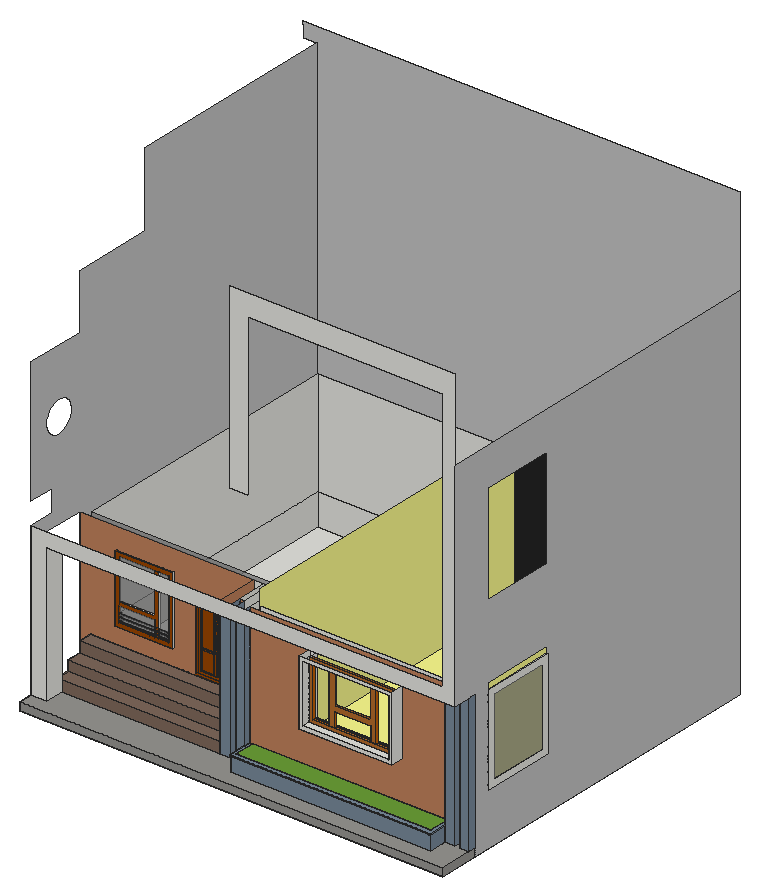
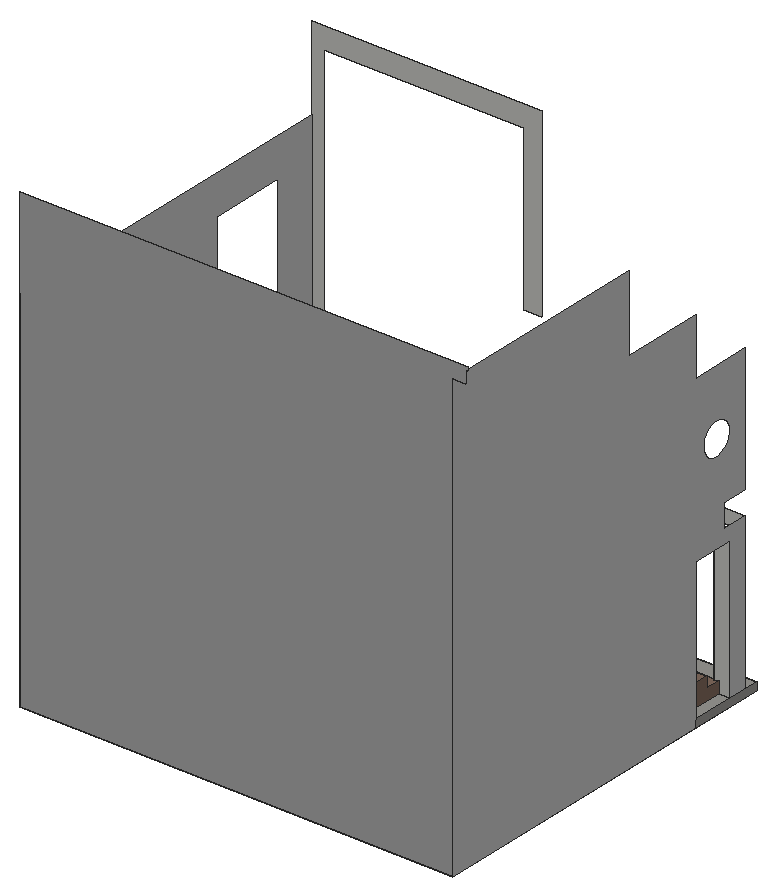
# SketchUp Ruby script. Lengths in inches.
U = 1.inch
M = Sketchup.active_model
def pt(a) = Geom::Point3d.new(a.map { |v| v * U })
def face(e, loops, mat)
  f = e.add_face(loops[0].map { |a| pt(a) })
  loops[1..].each { |l| e.add_face(l.map { |a| pt(a) }).erase! }
  f.material = f.back_material = mat if mat
  f
end
# faces: each face lists its corners as indices into pts; further lists are holes
def faces(e, pts, list, mat = nil) = list.each { |f| face(e, (f[0].is_a?(Array) ? f : [f]).map { |l| l.map { |i| pts[i] } }, mat) }
# xy, xz, yz: faces in a plane at the given z, y or x. An outline is a flat list of corners, or four numbers for a rectangle; further outlines are holes
def ring(l) = l.size == 4 ? [[l[0], l[1]], [l[2], l[1]], [l[2], l[3]], [l[0], l[3]]] : l.each_slice(2).to_a
def flat(e, list, mat, &to3) = list.each { |f| face(e, (f[0].is_a?(Array) ? f : [f]).map { |l| ring(l).map { |u, v| to3.(u, v) } }, mat) }
def xy(e, z, list, mat = nil) = flat(e, list, mat) { |x, y| [x, y, z] }
def xz(e, y, list, mat = nil) = flat(e, list, mat) { |x, z| [x, y, z] }
def yz(e, x, list, mat = nil) = flat(e, list, mat) { |y, z| [x, y, z] }
def lines(e, pts, list) = list.each { |a, b| e.add_line(pt(pts[a]), pt(pts[b])) }
# prism: a flat outline (further loops are holes) pulled along v
def prism(e, loops, v, mat = nil)
  f = face(e, loops, mat); d = Geom::Vector3d.new(v.map { |x| x * U })
  f.pushpull(f.normal.samedirection?(d) ? d.length : -d.length)
end
def box(e, o, s, mat = nil) = prism(e, [[o, [o[0] + s[0], o[1], o[2]], [o[0] + s[0], o[1] + s[1], o[2]], [o[0], o[1] + s[1], o[2]]]], [0, 0, s[2]], mat)
def at(x, y, z, deg = 0) = Geom::Transformation.translation(pt([x, y, z])) * Geom::Transformation.rotation(ORIGIN, Z_AXIS, deg.degrees)
def axes(o, x, y, z) = Geom::Transformation.new([*x, 0, *y, 0, *z, 0, *pt(o).to_a, 1])
def part(name) = M.definitions.add(name)
# library, detail: a bought-in or finely detailed component or shape, given as its bounding box
def library(name, o, s) = part(name).tap { |d| box(d.entities, o, s) }
def detail(e, o, s) = box(e.add_group.entities, o, s)
def put(e, d, t, mat = nil) = e.add_instance(d, t).tap { |i| i.material = mat if mat }
def group(e, t, mat = nil) = e.add_group.tap { |g| g.transformation = t; g.material = mat if mat }.entities
root = M.entities
M.materials.add("[0032_Moccasin]").color = [249, 249, 141]
M.materials.add("[0110_LightSlateGray]").color = [119, 130, 163]
M.materials.add("[0110_LightSlateGray]1").color = [119, 136, 153]
M.materials.add("[0131_Silver]").color = [192, 192, 192]
M.materials.add("[0132_LightGray]").color = [169, 169, 169]
M.materials.add("[0136_Charcoal]").color = [35, 35, 35]
M.materials.add("[Granite Brown]").color = [126, 104, 91]
M.materials.add("[Granite Light Gray]").color = [149, 148, 144]
M.materials.add("[Grass Dark Green]").color = [106, 157, 55]
M.materials.add("[Translucent Glass Gray]").color = [128, 128, 128]
M.materials["[Translucent Glass Gray]"].alpha = 0.68
M.materials.add("[Wood Bamboo]").color = [195, 96, 5]
M.materials.add("[Wood Bamboo]1").color = [177, 105, 43]
M.materials.add("[Wood Cherry Original]").color = [152, 68, 0]
M.materials.add("[Wood Veneer 02]").color = [190, 128, 91]
xy(root,0,[[15.875,0,495.875,420]])
xy(root,9,[[15.875,15.6875,24.875,36.73],[24.875,15.6875,33.875,36.73],[241.25,16.625,468.26,44.6875],[213.63,36.625,225.4375,84.25],[230.75,36.625,241.25,84.25],
  [468.26,36.625,480.0625,44.6875],[485.375,36.625,486.875,44.6875],[486.875,36.625,495.875,44.6875],[28.41,36.73,213.63,52.57],[225.4375,49.4375,230.75,84.25],
  [28.41,52.57,213.63,84.25],[24.875,90.25,241.25,411]])
xy(root,9,[[247.25,50.6875,486.875,411]],"[0032_Moccasin]")
xy(root,9,[[15.875,0,495.875,0,495.875,36.625,485.375,36.625,485.375,44.6875,480.0625,44.6875,480.0625,36.625,468.26,36.625,468.26,16.625,241.25,16.625,241.25,36.625,230.75,36.625,230.75,49.4375,225.4375,49.4375,225.4375,36.625,213.63,36.625,213.63,36.73,33.875,36.73,33.875,15.6875,15.875,15.6875],[15.875,36.73,28.41,84.25]],"[Granite Light Gray]")
xy(root,21,[[28.41,36.73,213.63,52.57]],"[Granite Brown]")
xy(root,25.5,[[240.75,16.125,240.75,36.625,241.25,36.625,241.25,16.625,468.26,16.625,468.26,36.625,468.76,36.625,468.76,16.125]],"[0110_LightSlateGray]1")
xy(root,27,[[240.75,16.125,468.76,16.125,468.76,36.625,468.26,36.625,468.26,44.6875,465.26,44.6875,465.26,20.625,244.25,20.625,244.25,44.6875,241.25,44.6875,241.25,36.625,240.75,36.625]],"[0110_LightSlateGray]1")
xy(root,27.0625,[[244.25,20.625,465.26,44.6875]],"[Grass Dark Green]")
xy(root,33,[[28.41,52.57,213.63,68.41]],"[Granite Brown]")
xy(root,45,[[28.41,68.41,213.63,84.25]],"[Granite Brown]")
xy(root,48,[[149.49,84.25,191.49,85.25]],"[Wood Cherry Original]")
xy(root,52.5,[[154,85.05,167.69,85.25],[173.29,85.05,186.99,85.25]])
xy(root,60,[[495.875,63.375,496.875,147.375]])
xy(root,64.51,[[57.9375,82.25,123.25,84.25]])
xy(root,67,[[495.875,70.375,496.875,140.375]])
xy(root,68.51,[[61.9375,82.25,103.25,84.25],[103.25,82.25,107.25,84.25],[107.25,82.25,119.25,84.25]])
xy(root,70.78,[[308.2,30.4375,413.0625,44.6875]])
xy(root,72.24,[[154,85.05,167.69,85.25],[173.29,85.05,186.99,85.25]],"[Wood Cherry Original]")
xy(root,74.59,[[312.01,30.4375,409.26,39.5625],[312.01,39.5625,409.26,43],[312.01,43,409.26,50.6875]])
xy(root,75.24,[[154,85.05,167.69,85.25],[173.29,85.05,186.99,85.25]])
xy(root,78.59,[[316.01,39.5625,334.01,43],[334.01,39.5625,340.01,40.5625],[381.26,39.5625,387.26,40.5625]],"[Wood Bamboo]")
xy(root,78.59,[[340.01,39.5625,381.26,43],[387.26,39.5625,405.26,43]],"[Wood Bamboo]1")
xz(root,0,[[15.875,0,495.875,9]],"[Granite Light Gray]")
xz(root,15.6875,[[15.875,9,33.875,9,33.875,165,495.875,165,495.875,503.875,241.25,503.875,241.25,298.5,261.37,298.5,261.37,479,482.9375,479,482.9375,180.75,15.875,180.75]])
xz(root,16.125,[[240.75,25.5,468.76,27]],"[0110_LightSlateGray]1")
xz(root,16.625,[[241.25,9,468.26,25.5]],"[0110_LightSlateGray]1")
xz(root,20.625,[[244.25,27,465.26,27.0625]],"[0110_LightSlateGray]")
xz(root,30.4375,[[[308.2,70.78,413.0625,144.4],[312.01,74.59,409.26,140.59]]])
xz(root,36.625,[[240.75,25.5,241.25,27],[468.26,25.5,468.76,27]])
xz(root,36.625,[[213.63,9,225.4375,165],[230.75,9,241.25,9,241.25,25.5,240.75,25.5,240.75,27,241.25,27,241.25,165,230.75,165],[468.26,9,480.0625,9,480.0625,165,468.26,165,468.26,27,468.76,27,468.76,25.5,468.26,25.5],[485.375,9,495.875,165]],"[0110_LightSlateGray]1")
xz(root,36.73,[[15.875,9,15.875,165,33.875,165,33.875,21,28.41,21,28.41,9],[28.41,9,33.875,21]])
xz(root,36.73,[[33.875,9,213.63,21]],"[Granite Brown]")
xz(root,39.5625,[[[312.01,74.59,409.26,140.59],[316.01,78.59,405.26,136.59]]],"[Wood Bamboo]1")
xz(root,40.5625,[[334.01,78.59,340.01,78.59,340.01,94.9,381.26,94.9,381.26,78.59,387.26,78.59,387.26,136.59,381.26,136.59,381.26,100.9,340.01,100.9,340.01,136.59,334.01,136.59]],"[Wood Bamboo]1")
xz(root,43,[[[312.01,74.59,409.26,140.59],[340.01,100.9,381.26,136.59],[387.26,78.59,405.26,136.59],[316.01,78.59,334.01,136.59],[340.01,78.59,381.26,94.9]]],"[Wood Bamboo]1")
xz(root,44.6875,[[241.25,9,468.26,9,468.26,27,465.26,27,465.26,27.0625,244.25,27.0625,244.25,27,241.25,27],[468.26,9,480.0625,165],[485.375,9,495.875,165]])
xz(root,44.6875,[[480.0625,9,485.375,165],[[241.25,27,244.25,27,244.25,27.0625,465.26,27.0625,465.26,27,468.26,27,468.26,165,241.25,165],[308.2,70.78,413.0625,144.4]]],"[Wood Veneer 02]")
xz(root,49.4375,[[225.4375,9,230.75,165]],"[Wood Veneer 02]")
xz(root,50.6875,[[247.25,9,486.875,45],[[247.25,45,486.875,165],[312.01,74.59,409.26,140.59]]])
xz(root,52.57,[[28.41,21,213.63,33]],"[Granite Brown]")
xz(root,63.375,[[495.875,60,496.875,162]])
xz(root,68.41,[[28.41,33,213.63,45]],"[Granite Brown]")
xz(root,70.375,[[495.875,67,496.875,155]])
xz(root,82.25,[[[57.9375,64.51,123.25,141.01],[61.9375,68.51,119.25,137.01]],[103.25,68.51,107.25,68.51,107.25,137.01,103.25,137.01,103.25,90.51,61.9375,90.51,61.9375,86.51,103.25,86.51]],"[Wood Cherry Original]")
xz(root,84.25,[[28.41,9,213.63,33],[213.63,9,225.4375,45],[225.4375,9,230.75,45],[230.75,9,241.25,45],[28.41,33,213.63,45],
  [213.63,45,225.4375,165],[225.4375,45,230.75,165],[230.75,45,241.25,165],[[57.9375,64.51,123.25,141.01],[61.9375,68.51,119.25,137.01]],[103.25,68.51,103.25,86.51,61.9375,86.51,61.9375,90.51,103.25,90.51,103.25,137.01,107.25,137.01,107.25,68.51]])
xz(root,84.25,[[[146.49,45,194.49,129],[149.49,48,191.49,126]]],"[Wood Cherry Original]")
xz(root,84.25,[[[15.875,9,28.41,9,28.41,45,146.49,45,146.49,129,194.49,129,194.49,45,213.63,45,213.63,165,15.875,165],[57.9375,64.51,123.25,141.01]]],"[Wood Veneer 02]")
xz(root,85.05,[[154,52.5,167.69,72.24],[173.29,52.5,186.99,72.24],[154,75.24,167.69,121.5],[173.29,75.24,186.99,121.5]],"[Wood Cherry Original]")
xz(root,85.25,[[[149.49,48,191.49,126],[152.5,51,188.49,123]],[152.5,51,154,52.5,154,72.24,152.5,73.74],[152.5,51,169.19,51,167.69,52.5,154,52.5],[169.19,51,169.19,73.74,167.69,72.24,167.69,52.5],[169.19,51,170.49,123],
  [170.49,51,171.79,123],[171.79,51,173.29,52.5,173.29,72.24,171.79,73.74],[171.79,51,188.49,51,186.99,52.5,173.29,52.5],[188.49,51,188.49,73.74,186.99,72.24,186.99,52.5],[154,72.24,167.69,72.24,169.19,73.74,152.5,73.74],
  [173.29,72.24,186.99,72.24,188.49,73.74,171.79,73.74],[152.5,73.74,154,75.24,154,121.5,152.5,123],[152.5,73.74,169.19,73.74,167.69,75.24,154,75.24],[169.19,73.74,169.19,123,167.69,121.5,167.69,75.24],[171.79,73.74,173.29,75.24,173.29,121.5,171.79,123],
  [171.79,73.74,188.49,73.74,186.99,75.24,173.29,75.24],[188.49,73.74,188.49,123,186.99,121.5,186.99,75.24]],"[Wood Cherry Original]")
xz(root,90.25,[[24.875,9,241.25,45]])
xz(root,90.25,[[24.875,45,241.25,165]],"[Translucent Glass Gray]")
xz(root,140.375,[[495.875,67,496.875,155]])
xz(root,147.375,[[495.875,60,496.875,162]])
xz(root,411,[[24.875,9,241.25,45],[241.25,9,247.25,45],[24.875,45,241.25,165],[241.25,45,247.25,165]])
xz(root,411,[[293.79,9,402.93,182]],"[0032_Moccasin]")
xz(root,411,[[247.25,9,293.79,182],[402.93,9,486.875,182]],"[0136_Charcoal]")
xz(root,420,[[15.875,0,15.875,494,2.0625,494,2.0625,507.4375,0,507.4375,0,511,495.875,511,495.875,0]],"[0131_Silver]")
yz(root,15.875,[[[84.25,0,84.25,165,36.73,165,36.73,9,15.6875,9,15.6875,180.75,44.6875,180.75,44.6875,205.89,15.6875,205.89,15.6875,347,84.25,347,84.25,410,176.25,410,176.25,494,420,494,420,0],[56.56,256.125,61.1875,257.12,65.4,259.27,68.91,262.45,71.48,266.42,72.93,270.92,73.17,275.65,72.18,280.27,70.02,284.49,66.85,288,62.87,290.57,58.37,292.02,53.64,292.26,49.02,291.26,44.81,289.11,41.3,285.93,38.73,281.96,37.27,277.46,37.04,272.73,38.03,268.11,40.19,263.89,43.36,260.38,47.33,257.82,51.83,256.36]]],"[0131_Silver]")
yz(root,15.875,[[0,0,84.25,9]],"[Granite Light Gray]")
yz(root,24.875,[[90.25,9,411,45],[90.25,45,411,165]])
yz(root,28.41,[[36.73,9,36.73,21,52.57,21,52.57,33,68.41,33,68.41,45,84.25,45,84.25,9]],"[Granite Brown]")
yz(root,33.875,[[15.6875,9,36.73,165]])
yz(root,57.9375,[[82.25,64.51,84.25,141.01]],"[Wood Cherry Original]")
yz(root,61.9375,[[[82.25,68.51,84.25,68.51,84.25,86.51,83.74,86.51,83.75,86.46,83.73,86.34,83.68,86.21,83.6,86.11,83.5,86.03,83.38,85.98,83.25,85.96,83.12,85.98,83,86.03,82.9,86.11,82.82,86.21,82.77,86.34,82.75,86.46,82.76,86.51,82.25,86.51],[83.25,69.96,83.12,69.98,83,70.03,82.9,70.11,82.82,70.21,82.77,70.34,82.75,70.46,82.77,70.59,82.82,70.71,82.9,70.82,83,70.9,83.12,70.95,83.25,70.96,83.38,70.95,83.5,70.9,83.6,70.82,83.68,70.71,83.73,70.59,83.75,70.46,83.73,70.34,83.68,70.21,83.6,70.11,83.5,70.03,83.38,69.98]]],"[Wood Cherry Original]")
yz(root,103.25,[[82.25,68.51,84.25,86.51]],"[Wood Cherry Original]")
yz(root,107.25,[[82.25,68.51,84.25,137.01]])
yz(root,119.25,[[[82.25,68.51,84.25,137.01],[83.25,69.96,83.38,69.98,83.5,70.03,83.6,70.11,83.68,70.21,83.73,70.34,83.75,70.46,83.73,70.59,83.68,70.71,83.6,70.82,83.5,70.9,83.38,70.95,83.25,70.96,83.12,70.95,83,70.9,82.9,70.82,82.82,70.71,82.77,70.59,82.75,70.46,82.77,70.34,82.82,70.21,82.9,70.11,83,70.03,83.12,69.98]]],"[Wood Cherry Original]")
yz(root,123.25,[[82.25,64.51,84.25,141.01]])
yz(root,149.49,[[84.25,48,85.25,126]],"[Wood Cherry Original]")
yz(root,154,[[85.05,52.5,85.25,72.24],[85.05,75.24,85.25,121.5]])
yz(root,167.69,[[85.05,52.5,85.25,72.24],[85.05,75.24,85.25,121.5]],"[Wood Cherry Original]")
yz(root,173.29,[[85.05,52.5,85.25,72.24],[85.05,75.24,85.25,121.5]],"[Wood Cherry Original]")
yz(root,186.99,[[85.05,52.5,85.25,72.24],[85.05,75.24,85.25,121.5]])
yz(root,191.49,[[84.25,48,85.25,126]],"[Wood Cherry Original]")
yz(root,213.63,[[36.625,9,36.73,21],[36.73,9,36.73,21,52.57,21,52.57,33,68.41,33,68.41,45,84.25,45,84.25,9]])
yz(root,213.63,[[36.625,21,36.625,165,84.25,165,84.25,45,68.41,45,68.41,33,52.57,33,52.57,21]],"[Wood Veneer 02]")
yz(root,225.4375,[[49.4375,9,84.25,165]])
yz(root,225.4375,[[36.625,9,49.4375,165]],"[0110_LightSlateGray]1")
yz(root,230.75,[[49.4375,9,84.25,165]])
yz(root,230.75,[[36.625,9,49.4375,165]],"[0110_LightSlateGray]1")
yz(root,240.75,[[16.125,25.5,36.625,27]],"[0110_LightSlateGray]")
yz(root,241.25,[[36.625,9,44.6875,27],[44.6875,9,84.25,165],[90.25,9,411,45],[90.25,45,411,165]])
yz(root,241.25,[[16.625,9,36.625,25.5]],"[0110_LightSlateGray]")
yz(root,241.25,[[36.625,27,44.6875,165]],"[0110_LightSlateGray]1")
yz(root,244.25,[[20.625,27,44.6875,27.0625]],"[0110_LightSlateGray]")
yz(root,247.25,[[50.6875,9,411,182]],"[0032_Moccasin]")
yz(root,308.2,[[30.4375,70.78,44.6875,144.4]])
yz(root,312.01,[[30.4375,74.59,39.5625,140.59],[39.5625,74.59,43,140.59],[43,74.59,50.6875,140.59]])
yz(root,316.01,[[[39.5625,78.59,43,136.59],[41.28,79.71,41.15,79.73,41.03,79.78,40.93,79.86,40.85,79.96,40.8,80.08,40.78,80.21,40.8,80.34,40.85,80.46,40.93,80.57,41.03,80.65,41.15,80.7,41.28,80.71,41.41,80.7,41.53,80.65,41.63,80.57,41.71,80.46,41.76,80.34,41.78,80.21,41.76,80.08,41.71,79.96,41.63,79.86,41.53,79.78,41.41,79.73]]],"[Wood Bamboo]")
yz(root,334.01,[[40.5625,78.59,43,136.59]],"[Wood Bamboo]1")
yz(root,340.01,[[40.5625,78.59,43,94.9]],"[Wood Bamboo]")
yz(root,381.26,[[40.5625,78.59,43,94.9]],"[Wood Bamboo]1")
yz(root,387.26,[[40.5625,78.59,43,136.59]],"[Wood Bamboo]")
yz(root,405.26,[[[39.5625,78.59,43,136.59],[41.28,79.71,41.41,79.73,41.53,79.78,41.63,79.86,41.71,79.96,41.76,80.08,41.78,80.21,41.76,80.34,41.71,80.46,41.63,80.57,41.53,80.65,41.41,80.7,41.28,80.71,41.15,80.7,41.03,80.65,40.93,80.57,40.85,80.46,40.8,80.34,40.78,80.21,40.8,80.08,40.85,79.96,40.93,79.86,41.03,79.78,41.15,79.73]]],"[Wood Bamboo]1")
yz(root,409.26,[[30.4375,74.59,39.5625,140.59],[39.5625,74.59,43,140.59],[43,74.59,50.6875,140.59]])
yz(root,413.0625,[[30.4375,70.78,44.6875,144.4]])
yz(root,465.26,[[20.625,27,44.6875,27.0625]],"[0110_LightSlateGray]")
yz(root,468.26,[[36.625,9,44.6875,27]])
yz(root,468.26,[[36.625,27,44.6875,165]],"[0110_LightSlateGray]")
yz(root,468.26,[[16.625,9,36.625,25.5]],"[0110_LightSlateGray]1")
yz(root,468.76,[[16.125,25.5,36.625,27]],"[0110_LightSlateGray]1")
yz(root,480.0625,[[36.625,9,44.6875,165]],"[0110_LightSlateGray]1")
yz(root,485.375,[[36.625,9,44.6875,165]],"[0110_LightSlateGray]")
yz(root,486.875,[[50.6875,9,411,182]],"[0032_Moccasin]")
yz(root,495.875,[[[63.375,60,147.375,162],[70.375,67,140.375,155]]])
yz(root,495.875,[[36.625,9,44.6875,165]],"[0110_LightSlateGray]1")
yz(root,495.875,[[[44.6875,0,420,0,420,410,15.6875,410,15.6875,165,44.6875,165],[63.375,253,147.375,367],[63.375,60,147.375,169]]],"[0131_Silver]")
yz(root,495.875,[[0,0,44.6875,9]],"[Granite Light Gray]")
yz(root,495.875,[[70.375,67,140.375,155]],"[Translucent Glass Gray]")
yz(root,496.875,[[[63.375,60,147.375,162],[70.375,67,140.375,155]]])
p = [[119.25,83,70.03],[119.25,82.9,70.11],[61.9375,82.9,70.11],[61.9375,83,70.03],[119.25,83.12,69.98],[61.9375,83.12,69.98],
  [119.25,83.25,69.96],[61.9375,83.25,69.96],[119.25,83.38,69.98],[61.9375,83.38,69.98],[119.25,83.5,70.03],[61.9375,83.5,70.03],
  [119.25,83.6,70.11],[61.9375,83.6,70.11],[119.25,82.82,70.21],[61.9375,82.82,70.21],[119.25,83.68,70.21],[61.9375,83.68,70.21],
  [119.25,82.77,70.34],[61.9375,82.77,70.34],[119.25,83.73,70.34],[61.9375,83.73,70.34],[119.25,82.75,70.46],[61.9375,82.75,70.46],
  [119.25,83.75,70.46],[61.9375,83.75,70.46],[119.25,82.77,70.59],[61.9375,82.77,70.59],[119.25,83.73,70.59],[61.9375,83.73,70.59],
  [119.25,82.82,70.71],[61.9375,82.82,70.71],[119.25,83.68,70.71],[61.9375,83.68,70.71],[119.25,82.9,70.82],[61.9375,82.9,70.82],
  [119.25,83.6,70.82],[61.9375,83.6,70.82],[119.25,83,70.9],[61.9375,83,70.9],[119.25,83.5,70.9],[61.9375,83.5,70.9],
  [119.25,83.12,70.95],[61.9375,83.12,70.95],[119.25,83.25,70.96],[61.9375,83.25,70.96],[119.25,83.38,70.95],[61.9375,83.38,70.95],
  [119.25,83,74.03],[119.25,82.9,74.11],[61.9375,82.9,74.11],[61.9375,83,74.03],[119.25,83.12,73.98],[61.9375,83.12,73.98],
  [119.25,83.25,73.96],[61.9375,83.25,73.96],[119.25,83.38,73.98],[61.9375,83.38,73.98],[119.25,83.5,74.03],[61.9375,83.5,74.03],
  [119.25,83.6,74.11],[61.9375,83.6,74.11],[119.25,82.82,74.21],[61.9375,82.82,74.21],[119.25,83.68,74.21],[61.9375,83.68,74.21],
  [119.25,82.77,74.34],[61.9375,82.77,74.34],[119.25,83.73,74.34],[61.9375,83.73,74.34],[119.25,82.75,74.46],[61.9375,82.75,74.46],
  [119.25,83.75,74.46],[61.9375,83.75,74.46],[119.25,82.77,74.59],[61.9375,82.77,74.59],[119.25,83.73,74.59],[61.9375,83.73,74.59],
  [119.25,82.82,74.71],[61.9375,82.82,74.71],[119.25,83.68,74.71],[61.9375,83.68,74.71],[119.25,82.9,74.82],[61.9375,82.9,74.82],
  [119.25,83.6,74.82],[61.9375,83.6,74.82],[119.25,83,74.9],[61.9375,83,74.9],[119.25,83.5,74.9],[61.9375,83.5,74.9],
  [119.25,83.12,74.95],[61.9375,83.12,74.95],[119.25,83.25,74.96],[61.9375,83.25,74.96],[119.25,83.38,74.95],[61.9375,83.38,74.95],
  [119.25,83,78.03],[119.25,82.9,78.11],[61.9375,82.9,78.11],[61.9375,83,78.03],[119.25,83.12,77.98],[61.9375,83.12,77.98],
  [119.25,83.25,77.96],[61.9375,83.25,77.96],[119.25,83.38,77.98],[61.9375,83.38,77.98],[119.25,83.5,78.03],[61.9375,83.5,78.03],
  [119.25,83.6,78.11],[61.9375,83.6,78.11],[119.25,82.82,78.21],[61.9375,82.82,78.21],[119.25,83.68,78.21],[61.9375,83.68,78.21],
  [119.25,82.77,78.34],[61.9375,82.77,78.34],[119.25,83.73,78.34],[61.9375,83.73,78.34],[119.25,82.75,78.46],[61.9375,82.75,78.46],
  [119.25,83.75,78.46],[61.9375,83.75,78.46],[119.25,82.77,78.59],[61.9375,82.77,78.59],[119.25,83.73,78.59],[61.9375,83.73,78.59],
  [119.25,82.82,78.71],[61.9375,82.82,78.71],[119.25,83.68,78.71],[61.9375,83.68,78.71],[119.25,82.9,78.82],[61.9375,82.9,78.82],
  [119.25,83.6,78.82],[61.9375,83.6,78.82],[119.25,83,78.9],[61.9375,83,78.9],[119.25,83.5,78.9],[61.9375,83.5,78.9],
  [119.25,83.12,78.95],[61.9375,83.12,78.95],[119.25,83.25,78.96],[61.9375,83.25,78.96],[119.25,83.38,78.95],[61.9375,83.38,78.95],
  [28.41,68.41,21],[213.63,68.41,21]]
faces(root,p,[[0,1,2,3],[4,0,3,5],[6,4,5,7],[8,6,7,9],[10,8,9,11],[12,10,11,13],[1,14,15,2],[16,12,13,17],
  [14,18,19,15],[20,16,17,21],[18,22,23,19],[24,20,21,25],[22,26,27,23],[28,24,25,29],[26,30,31,27],[32,28,29,33],
  [30,34,35,31],[36,32,33,37],[34,38,39,35],[40,36,37,41],[38,42,43,39],[42,44,45,43],[44,46,47,45],[46,40,41,47],
  [48,49,50,51],[52,48,51,53],[54,52,53,55],[56,54,55,57],[58,56,57,59],[60,58,59,61],[49,62,63,50],[64,60,61,65],
  [62,66,67,63],[68,64,65,69],[66,70,71,67],[72,68,69,73],[70,74,75,71],[76,72,73,77],[74,78,79,75],[80,76,77,81],
  [78,82,83,79],[84,80,81,85],[82,86,87,83],[88,84,85,89],[86,90,91,87],[90,92,93,91],[92,94,95,93],[94,88,89,95],
  [96,97,98,99],[100,96,99,101],[102,100,101,103],[104,102,103,105],[106,104,105,107],[108,106,107,109],[97,110,111,98],[112,108,109,113],
  [110,114,115,111],[116,112,113,117],[114,118,119,115],[120,116,117,121],[118,122,123,119],[124,120,121,125],[122,126,127,123],[128,124,125,129],
  [126,130,131,127],[132,128,129,133],[130,134,135,131],[136,132,133,137],[134,138,139,135],[138,140,141,139],[140,142,143,141],[142,136,137,143]],"[0132_LightGray]")
lines(root,p,[[144,145]])
